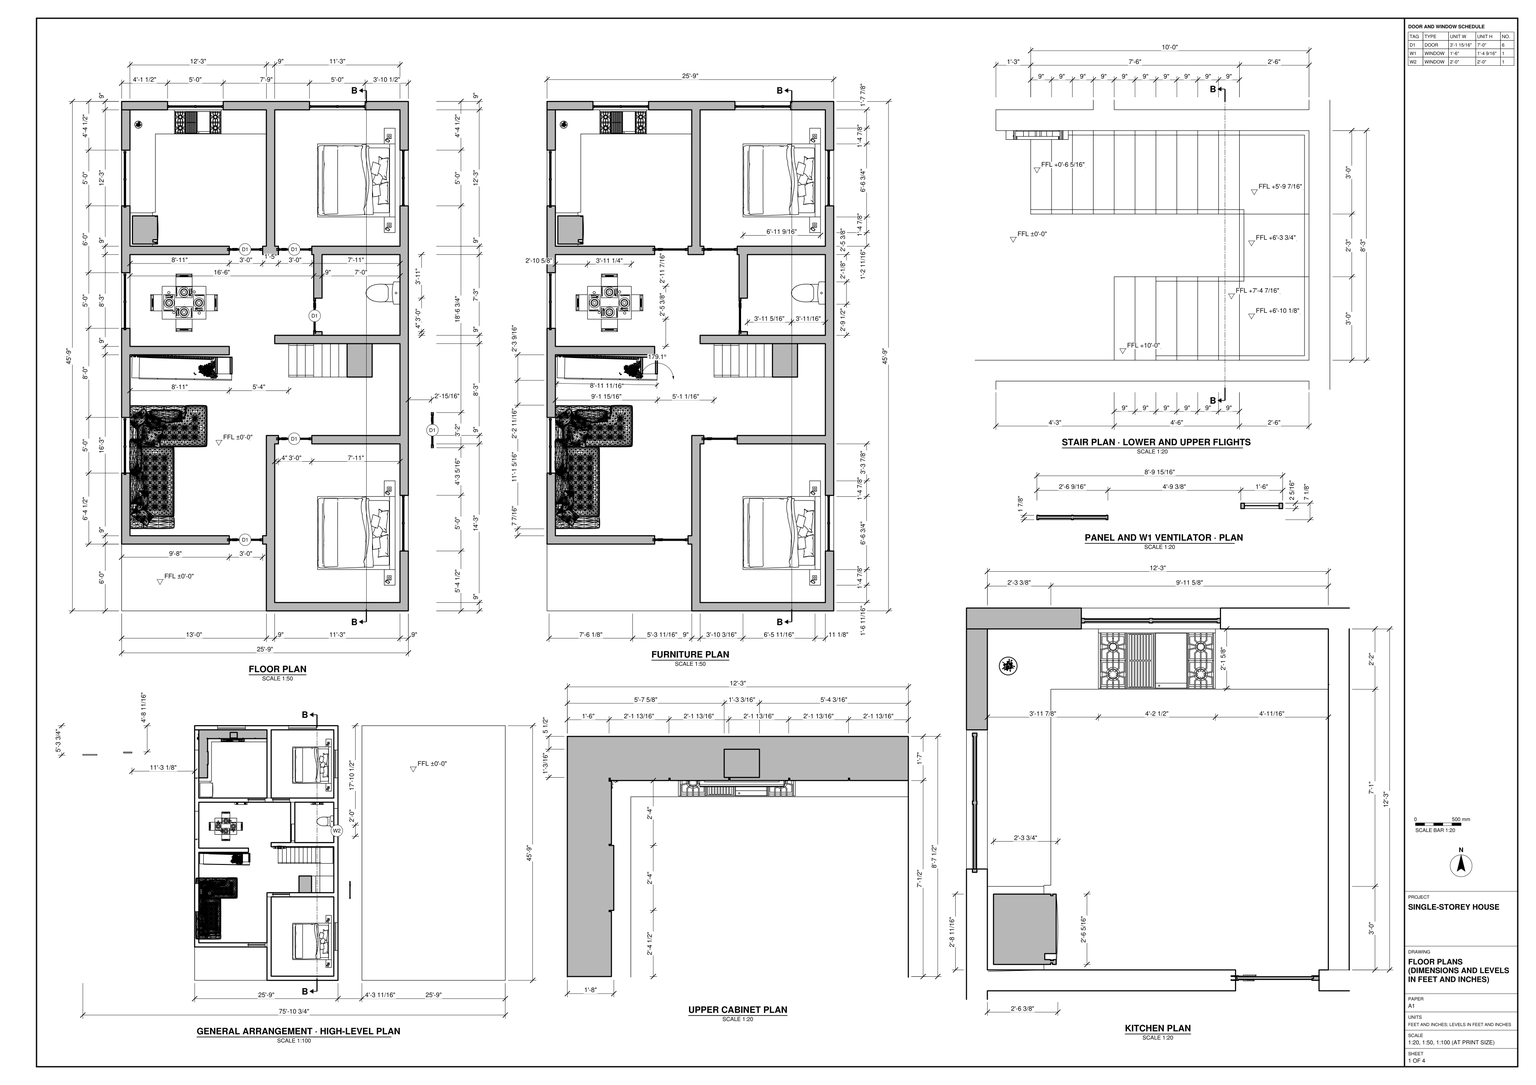
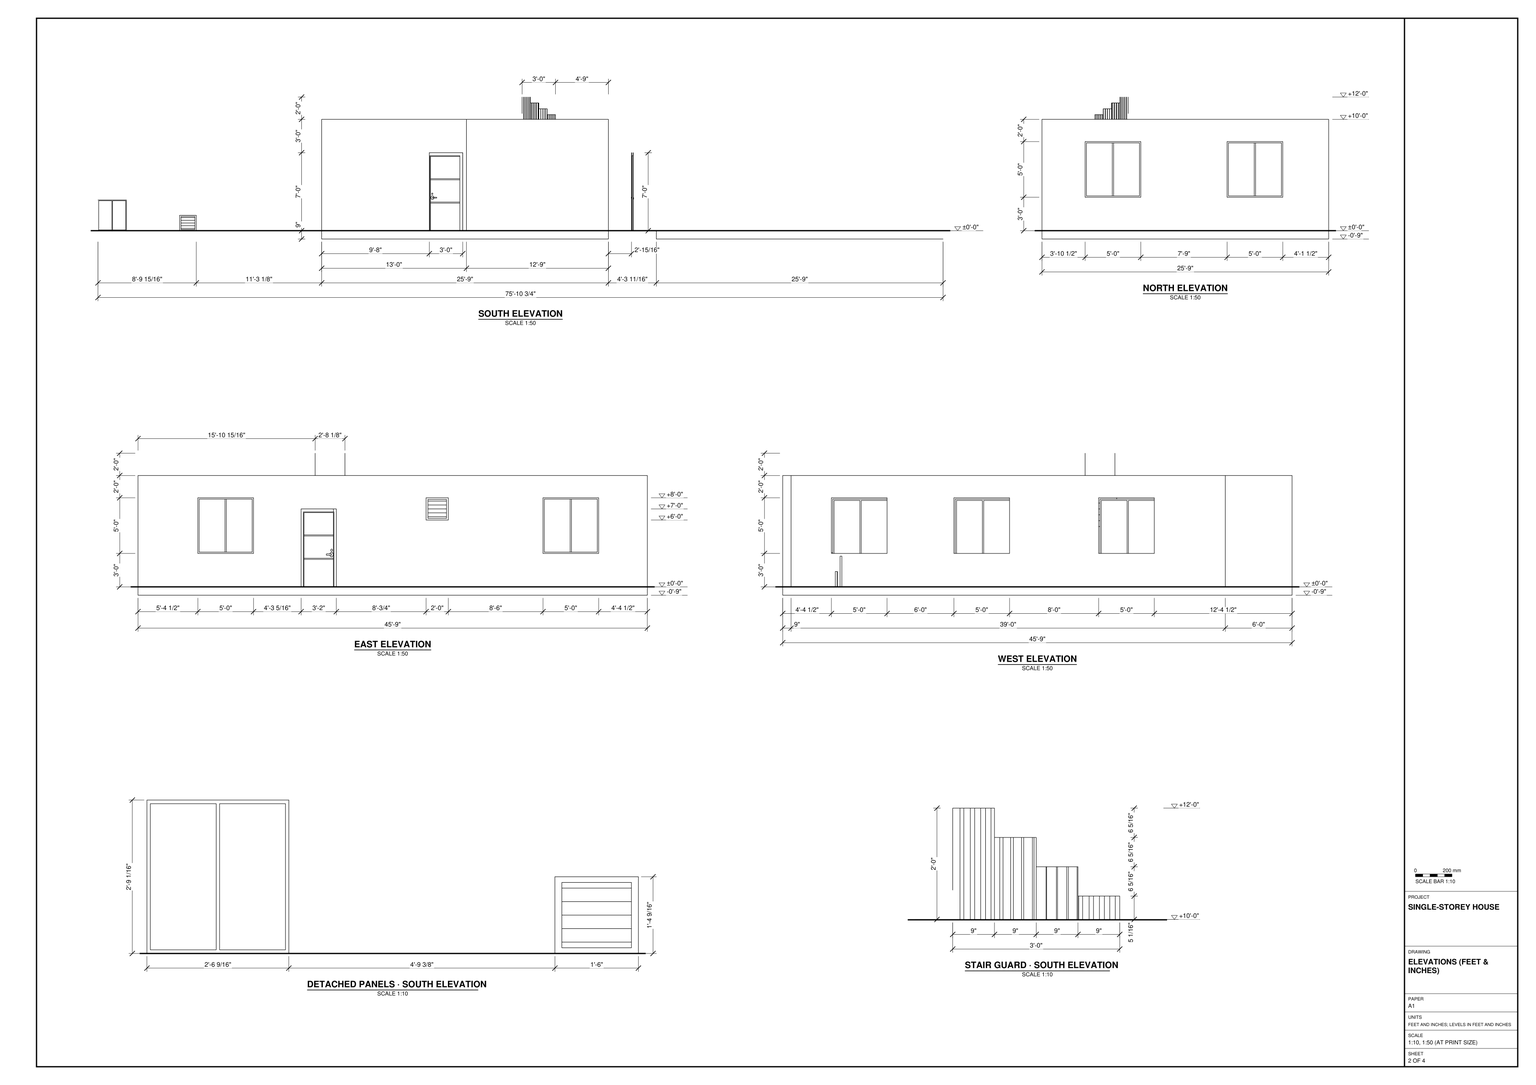
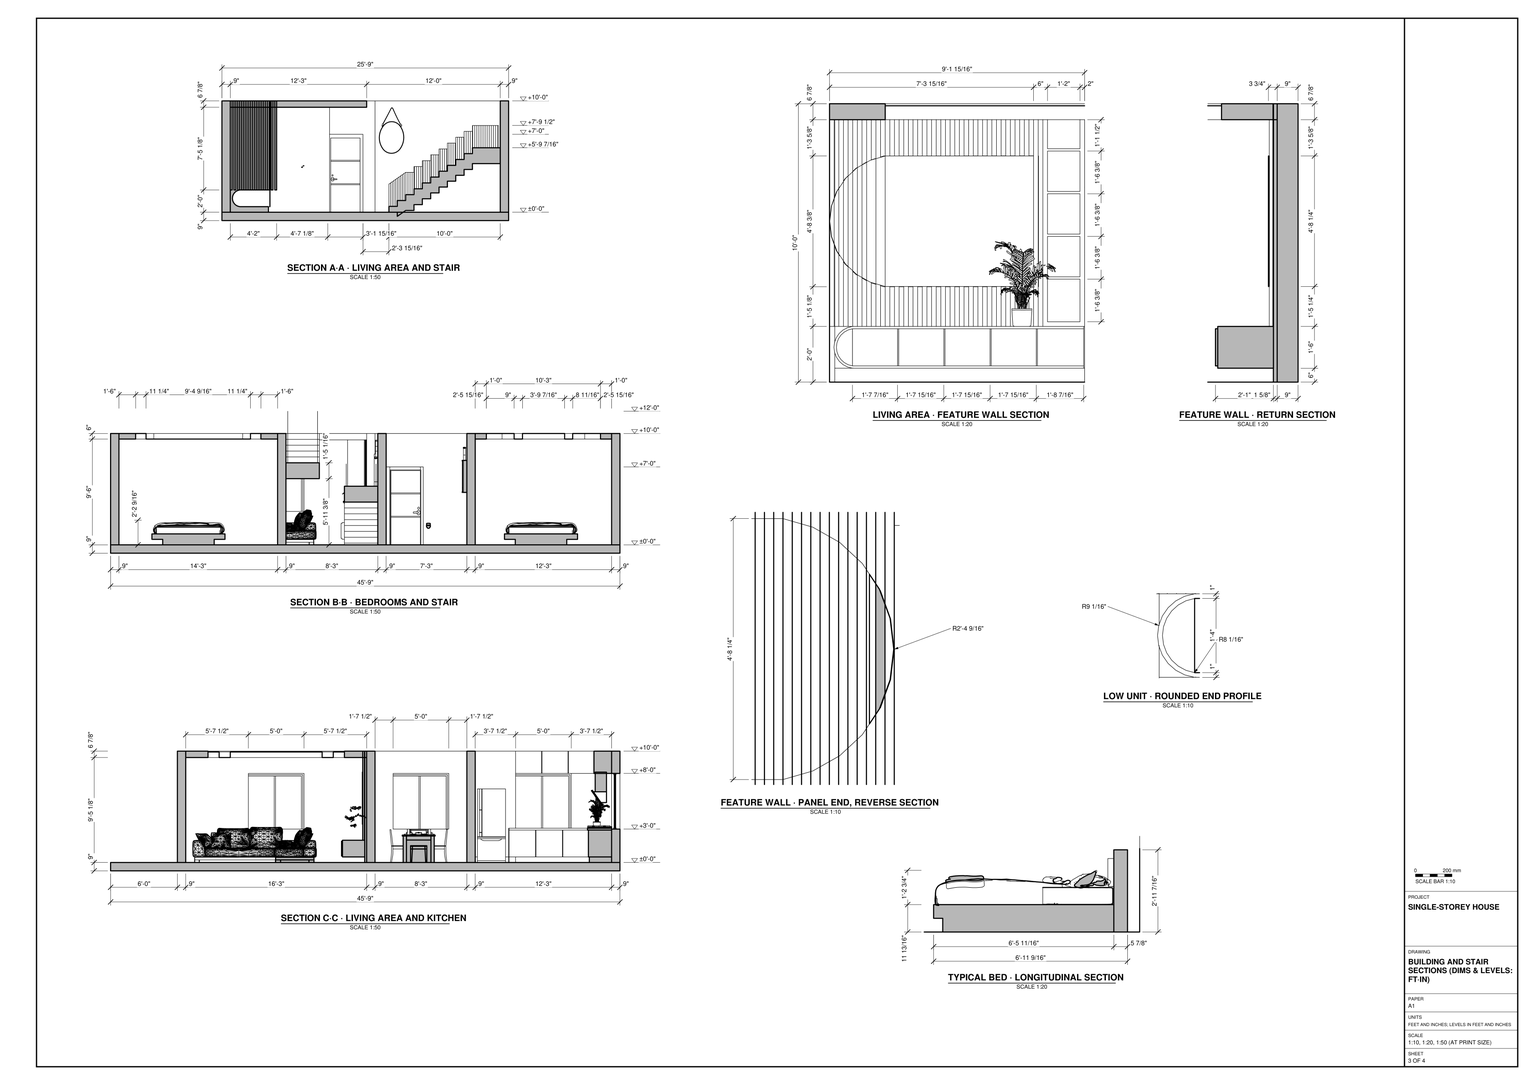
Build the single-storey house in SketchUp from task_files/diagram_01.pdf. Work in feet and inches. Set the ground-floor finished level to ±0'-0". The complete arrangement measures 75'-10 3/4" along X, 45'-9" along Y and 10'-9" along Z. The house itself is 25'-9" wide. Use the general arrangement plan to position the separate rectangular slab and detached units rather than widening the house to fill the overall extent.

Form the recessed southern entrance beside the projecting bedroom. Use the wall thicknesses shown on the floor plan, cut the door and window openings, and follow the sections for the slabs and roof. Place the kitchen in the northwest corner, with dining space immediately south of it and the living area by the entrance. Place the bedrooms at opposite ends of the east side, with the toilet compartment and return stair between them. Model both stair flights, the turning landing and the stepped guard.

Fit the kitchen with its L-shaped counter, upper cabinets, cooktop and hood. Use the furniture plan for the platform beds, four-place dining set and corner sofa. Reproduce the living-area feature wall, including the rounded panel end, low storage unit and side shelving. Decor and loose items may be any suitable library components. Keep shell elements and each furniture or joinery piece in separate groups or components, and use components for repeated parts. Save one SketchUp model as output_files/furnished_single_storey_house_with_a_return_stair.skp.

# SketchUp Ruby script. Lengths in inches.
U = 1.inch
M = Sketchup.active_model
def pt(a) = Geom::Point3d.new(a.map { |v| v * U })
def face(e, loops, mat)
  f = e.add_face(loops[0].map { |a| pt(a) })
  loops[1..].each { |l| e.add_face(l.map { |a| pt(a) }).erase! }
  f.material = f.back_material = mat if mat
  f
end
# faces: each face lists its corners as indices into pts; further lists are holes
def faces(e, pts, list, mat = nil) = list.each { |f| face(e, (f[0].is_a?(Array) ? f : [f]).map { |l| l.map { |i| pts[i] } }, mat) }
# xy, xz, yz: faces in a plane at the given z, y or x. An outline is a flat list of corners, or four numbers for a rectangle; further outlines are holes
def ring(l) = l.size == 4 ? [[l[0], l[1]], [l[2], l[1]], [l[2], l[3]], [l[0], l[3]]] : l.each_slice(2).to_a
def flat(e, list, mat, &to3) = list.each { |f| face(e, (f[0].is_a?(Array) ? f : [f]).map { |l| ring(l).map { |u, v| to3.(u, v) } }, mat) }
def xy(e, z, list, mat = nil) = flat(e, list, mat) { |x, y| [x, y, z] }
def xz(e, y, list, mat = nil) = flat(e, list, mat) { |x, z| [x, y, z] }
def yz(e, x, list, mat = nil) = flat(e, list, mat) { |y, z| [x, y, z] }
def lines(e, pts, list) = list.each { |a, b| e.add_line(pt(pts[a]), pt(pts[b])) }
# prism: a flat outline (further loops are holes) pulled along v
def prism(e, loops, v, mat = nil)
  f = face(e, loops, mat); d = Geom::Vector3d.new(v.map { |x| x * U })
  f.pushpull(f.normal.samedirection?(d) ? d.length : -d.length)
end
def box(e, o, s, mat = nil) = prism(e, [[o, [o[0] + s[0], o[1], o[2]], [o[0] + s[0], o[1] + s[1], o[2]], [o[0], o[1] + s[1], o[2]]]], [0, 0, s[2]], mat)
def at(x, y, z, deg = 0) = Geom::Transformation.translation(pt([x, y, z])) * Geom::Transformation.rotation(ORIGIN, Z_AXIS, deg.degrees)
def axes(o, x, y, z) = Geom::Transformation.new([*x, 0, *y, 0, *z, 0, *pt(o).to_a, 1])
def part(name) = M.definitions.add(name)
# library, detail: a bought-in or finely detailed component or shape, given as its bounding box
def library(name, o, s) = part(name).tap { |d| box(d.entities, o, s) }
def detail(e, o, s) = box(e.add_group.entities, o, s)
def put(e, d, t, mat = nil) = e.add_instance(d, t).tap { |i| i.material = mat if mat }
def group(e, t, mat = nil) = e.add_group.tap { |g| g.transformation = t; g.material = mat if mat }.entities
root = M.entities
M.materials.add("[0035_Tan]").color = [210, 180, 140]
M.materials.add("[0036_BurlyWood]").color = [222, 184, 135]
M.materials.add("[0042_Sienna]").color = [160, 82, 45]
M.materials.add("[0049_Beige]").color = [245, 245, 220]
M.materials.add("[0054_LightYellow]").color = [255, 255, 224]
M.materials.add("[0110_LightSlateGray]").color = [119, 136, 153]
M.materials.add("[0111_SlateGray]").color = [112, 128, 144]
M.materials.add("[0119_RosyBrown]").color = [188, 143, 143]
M.materials.add("[Carrera Marble]").color = [207, 207, 207]
M.materials["[Carrera Marble]"].alpha = 0.99
M.materials.add("[Color M09]").color = [0, 0, 0]
M.materials.add("[Color_008]").color = [30, 30, 30]
M.materials.add("[Color_009]").color = [0, 0, 0]
M.materials.add("[Translucent Glass Gray]").color = [128, 128, 128]
M.materials["[Translucent Glass Gray]"].alpha = 0.5
M.materials.add("[Translucent Glass Tinted]1").color = [7, 201, 240]
M.materials["[Translucent Glass Tinted]1"].alpha = 0.48
M.materials.add("[Translucent_Glass_Gray]").color = [128, 128, 128]
M.materials["[Translucent_Glass_Gray]"].alpha = 0.5
M.materials.add("[Wood Cherry Original]").color = [152, 86, 42]
M.materials.add("[Wood Floor Parquet]").color = [145, 89, 39]
M.materials.add("[Wood Floor]").color = [155, 105, 61]
c1 = library("main+door",[0,-0.79,0],[47.24,7.88,82.68])
c2 = part("ventilator")
g1 = group(c2.entities,at(0,0,0))
xy(g1,0,[[0,0,24,1],[0,1,24,6.83]],"[Wood Floor Parquet]")
xy(g1,1.75,[[2,0,22,6.83]],"[Wood Floor Parquet]")
xy(g1,21.87,[[2,0,22,6.83]],"[Wood Cherry Original]")
xy(g1,23.62,[[0,0,24,1],[0,1,24,6.83]],"[Wood Floor Parquet]")
xz(g1,0,[[[0,0,24,23.62],[2,1.75,22,21.87]]],"[Wood Floor Parquet]")
xz(g1,6.83,[[[0,0,24,23.62],[2,1.75,22,21.87]]],"[Wood Cherry Original]")
yz(g1,0,[[0,0,1,23.62],[1,0,6.83,23.62]],"[Wood Floor Parquet]")
yz(g1,2,[[0,1.75,6.83,1.75,6.83,7.66,0,3.5],[0,3.5,6.83,7.66,6.83,11.8125,0,7.66],[0,7.66,6.83,11.8125,6.83,15.97,0,11.8125],[0,11.8125,6.83,15.97,6.83,20.12,0,15.97],[0,15.97,6.83,20.12,6.83,21.87,0,21.87]],"[Wood Floor Parquet]")
yz(g1,22,[[0,1.75,0,3.5,6.83,7.66,6.83,1.75],[0,3.5,0,7.66,6.83,11.8125,6.83,7.66],[0,7.66,0,11.8125,6.83,15.97,6.83,11.8125],[0,11.8125,0,15.97,6.83,20.12,6.83,15.97],[0,15.97,0,21.87,6.83,21.87,6.83,20.12]],"[Wood Floor Parquet]")
yz(g1,24,[[0,0,1,23.62],[1,0,6.83,23.62]],"[Wood Floor Parquet]")
p = [[2,0,3.5],[2,6.83,7.66],[22,6.83,7.66],[22,0,3.5],[2,6.83,11.8125],[2,0,7.66],
  [22,0,7.66],[22,6.83,11.8125],[2,0,11.8125],[2,6.83,15.97],[22,6.83,15.97],[22,0,11.8125],
  [2,6.83,20.12],[2,0,15.97],[22,0,15.97],[22,6.83,20.12]]
faces(g1,p,[[0,1,2,3],[4,5,6,7],[8,9,10,11]],"[Translucent Glass Tinted]1")
faces(g1,p,[[12,13,14,15]],"[Translucent Glass Gray]")
c3 = library("Component\#33",[0,0,0],[60.64,55.48,158.625])
c4 = library("Gas cooktop",[0,0,34.52],[24.41,48.07,2.63])
c5 = part("Inclined chimney")
g2 = group(c5.entities,at(1.97,2.08,2.89))
xy(g2,0,[[0,7.9,31.3,13.68]])
xy(g2,11.29,[[0,0,31.3,13.68]])
xz(g2,13.68,[[0,0,31.3,11.29]])
yz(g2,0,[[7.9,0,0,11.29,13.68,11.29,13.68,0]])
yz(g2,31.3,[[7.9,0,13.68,0,13.68,11.29,0,11.29]])
g3 = group(c5.entities,at(0,9.85,0.4))
g4 = group(g3,at(0,0.61,0.43))
prism(g4,[[[35.24,0,0],[35.24,-3.39,4.84],[35.24,-3.58,4.7],[35.24,-0.29,0]]],[-35.24,0,0])
g5 = group(g3,at(0,-3.21,4.99))
prism(g5,[[[35.24,-0.2,-0.12],[35.24,-3.16,5],[0,-3.16,5],[0,-0.2,-0.12]]],[0,0.2,0.12])
g6 = group(g3,at(0,-6.27,10.27))
prism(g6,[[[35.24,-0.19,-0.14],[35.24,-3.58,4.7],[0,-3.58,4.7],[0,-0.19,-0.14]]],[0,0.19,0.14])
g7 = group(g3,at(0,0.61,0.43))
prism(g7,[[[35.24,0,0],[35.24,0.96,0],[35.24,-9.52,14.96],[35.24,-10.16,14.51]]],[-35.24,0,0])
g8 = group(c5.entities,at(10.24,3.95,20.8))
box(g8,[0,0,-6.62],[14.76,11.8125,20.56])
g9 = group(c5.entities,at(0,10.1,0))
prism(g9,[[[35.24,0.46,0],[35.24,1.33,0],[35.24,1.33,0.83],[35.24,1.01,0.83],[35.24,0.37,0.83],[35.24,0,0.83],[35.24,0,0.64]]],[-35.24,0,0])
c6 = part("Inclined+chimney")
put(c6.entities,c5,at(34.17,38.97,0.69))
c7 = library("Double bed",[0,0,0],[83.59,112.46,35.43])
c8 = library("CS300DRT",[0,0,0],[27.18,17.85,30.31])
c9 = library("Senza",[-40.91,-66.2,-0.5],[133.3,90.15,38.26])
c10 = library("SKT_Nearly Natural 5' Kentia Palm Silk Tree",[-23.18,-17.61,0],[47.48,43.95,59.125])
c11 = library("DINING+TABLE_4+SEATER_+1200mm+x+900mm",[14.07,13.24,0],[72.26,62.1,36.02])
c12 = library("Round wall hanging",[0,0,0],[26.88,1.18,49.49])
c13 = part("Group\#2")
xy(c13.entities,0,[[0,0,82.68,1.18]],"[Color_009]")
xy(c13.entities,1.97,[[1.97,0.98,40.35,1.18],[42.32,0.98,80.71,1.18]])
xy(c13.entities,1.97,[[1.97,0,40.35,0.3],[42.32,0,80.71,0.3]],"[Color_009]")
xy(c13.entities,80.71,[[1.97,0,40.35,0.3],[42.32,0,80.71,0.3],[1.97,0.3,40.35,0.98],[42.32,0.3,80.71,0.98],[1.97,0.98,40.35,1.18],
  [42.32,0.98,80.71,1.18]])
xy(c13.entities,82.68,[[0,0,82.68,1.18]],"[Color_008]")
xz(c13.entities,0,[[[0,0,82.68,82.68],[1.97,1.97,40.35,80.71],[42.32,1.97,80.71,80.71]]],"[Color_009]")
xz(c13.entities,0.3,[[1.97,1.97,40.35,80.71],[42.32,1.97,80.71,80.71]],"[Translucent_Glass_Gray]")
xz(c13.entities,0.98,[[1.97,1.97,40.35,80.71],[42.32,1.97,80.71,80.71]],"[Translucent_Glass_Gray]")
xz(c13.entities,1.18,[[[0,0,82.68,82.68],[1.97,1.97,80.71,80.71]],[40.35,1.97,42.32,80.71]],"[Color_009]")
yz(c13.entities,0,[[0,0,1.18,82.68]],"[Color_009]")
yz(c13.entities,1.97,[[0.98,1.97,1.18,80.71]])
yz(c13.entities,1.97,[[0,1.97,0.3,80.71]],"[Color_009]")
yz(c13.entities,40.35,[[0,1.97,0.3,80.71],[0.98,1.97,1.18,80.71]],"[Color_009]")
yz(c13.entities,42.32,[[0,1.97,0.3,80.71],[0.98,1.97,1.18,80.71]])
yz(c13.entities,80.71,[[0,1.97,0.3,80.71],[0.98,1.97,1.18,80.71]],"[Color_009]")
yz(c13.entities,82.68,[[0,0,1.18,82.68]],"[Color_009]")
c14 = library("Group\#5",[0,0,-4.44],[120,99,148.43])
c15 = part("Square post")
box(c15.entities,[0,-2,0],[2,2,96])
c16 = part("Group\#8")
box(c16.entities,[0,-2,0],[2,2,96])
xy(root,0,[[274.45,516,397.07,540]])
xy(root,6,[[274.95,515,298.97,516],[299.47,515,323.5,516],[324,515,348.02,516],[348.52,515,372.55,516],[373.05,515,396.87,516]])
xy(root,34.9375,[[274.95,515,298.97,515,298.97,516,299.47,516,299.47,515,323.5,515,323.5,516,324,516,324,515,348.02,515,348.02,516,348.52,516,348.52,515,372.55,515,372.55,516,373.05,516,373.05,515,396.87,515,396.87,516,397.07,516,397.07,540,274.45,540,274.45,516,274.95,516]])
xy(root,96,[[250.07,436.5,250.07,540,268.07,540,268.07,520.69,269.07,520.69,269.07,493.5,268.07,493.5,268.07,493,270.07,493,270.07,465,268.07,465,268.07,464.5,269.07,464.5,269.07,436.5],[268.57,521,268.57,522,268.07,522,268.07,540,397.07,540,397.07,521,371.77,521,371.77,522,371.27,522,371.27,521,345.97,521,345.97,522,345.47,522,345.47,521,320.17,521,320.17,522,319.67,522,319.67,521,294.37,521,294.37,522,293.87,522,293.87,521]])
xy(root,120,[[250.07,436.5,269.07,436.5,269.07,464.5,268.07,464.5,268.07,465,270.07,465,270.07,493,268.07,493,268.07,493.5,269.07,493.5,269.07,520.69,268.07,520.69,268.07,540,250.07,540],[268.57,521,293.87,521,293.87,522,294.37,522,294.37,521,319.67,521,319.67,522,320.17,522,320.17,521,345.47,521,345.47,522,345.97,522,345.97,521,371.27,521,371.27,522,371.77,522,371.77,521,397.07,521,397.07,540,268.07,540,268.07,522,268.57,522]],"[Wood Floor]")
xz(root,436.5,[[250.07,96,269.07,120]],"[Wood Floor]")
xz(root,464.5,[[268.07,96,269.07,120]],"[Wood Floor]")
xz(root,465,[[268.07,96,270.07,120]],"[Wood Floor]")
xz(root,493,[[268.07,96,270.07,120]],"[Wood Floor]")
xz(root,493.5,[[268.07,96,269.07,120]],"[Wood Floor]")
xz(root,515,[[274.95,6,298.97,34.9375],[299.47,6,323.5,34.9375],[324,6,348.02,34.9375],[348.52,6,372.55,34.9375],[373.05,6,396.87,34.9375]],"[Wood Floor]")
xz(root,516,[[274.45,0,274.95,34.9375],[274.95,0,397.07,0,397.07,34.9375,396.87,34.9375,396.87,6,373.05,6,373.05,34.9375,372.55,34.9375,372.55,6,348.52,6,348.52,34.9375,348.02,34.9375,348.02,6,324,6,324,34.9375,323.5,34.9375,323.5,6,299.47,6,299.47,34.9375,298.97,34.9375,298.97,6,274.95,6],[397.07,0,397.57,34.9375]])
xz(root,520.69,[[268.07,96,269.07,120]],"[Wood Floor]")
xz(root,521,[[268.57,96,293.87,120],[294.37,96,319.67,120],[320.17,96,345.47,120],[345.97,96,371.27,120],[371.77,96,397.07,120]],"[Wood Floor]")
xz(root,522,[[268.07,96,268.57,120],[293.87,96,294.37,120],[319.67,96,320.17,120],[345.47,96,345.97,120],[371.27,96,371.77,120]])
xz(root,540,[[274.45,0,397.07,34.9375]])
yz(root,250.07,[[436.5,96,540,120]])
yz(root,268.07,[[464.5,96,465,120],[493,96,493.5,120],[520.69,96,522,120]],"[Wood Floor]")
yz(root,268.57,[[521,96,522,120]])
yz(root,269.07,[[436.5,96,464.5,120],[493.5,96,520.69,120]],"[Wood Floor]")
yz(root,270.07,[[465,96,493,120]],"[Wood Floor]")
yz(root,274.45,[[516,0,540,34.9375]])
yz(root,274.95,[[515,6,516,34.9375]])
yz(root,293.87,[[521,96,522,120]])
yz(root,294.37,[[521,96,522,120]])
yz(root,298.97,[[515,6,516,34.9375]])
yz(root,299.47,[[515,6,516,34.9375]])
yz(root,319.67,[[521,96,522,120]])
yz(root,320.17,[[521,96,522,120]])
yz(root,323.5,[[515,6,516,34.9375]])
yz(root,324,[[515,6,516,34.9375]])
yz(root,345.47,[[521,96,522,120]])
yz(root,345.97,[[521,96,522,120]])
yz(root,348.02,[[515,6,516,34.9375]])
yz(root,348.52,[[515,6,516,34.9375]])
yz(root,371.27,[[521,96,522,120]])
yz(root,371.77,[[521,96,522,120]])
yz(root,372.55,[[515,6,516,34.9375]])
yz(root,373.05,[[515,6,516,34.9375]])
yz(root,396.87,[[515,6,516,34.9375]])
yz(root,397.07,[[516,0,540,34.9375],[521,96,540,120]])
# 242 loose lines left out
put(root,c1,axes([574.98,213.76,0],[0,-0.80367,0],[0.33,0,0],[0,0,1.016]))
put(root,c2,axes([87.9375,490.01,0],[0.75,0,0],[0,0.34,0],[0,0,0.7]))
put(root,c3,axes([280.47,395.36,0],[0,0.5,0],[-0.5,0,0],[0,0,0.5]))
put(root,c4,axes([297.92,540,0.69],[0,-1.05,0],[1.05,0,0],[0,0,1.05]))
put(root,c6,axes([271.95,478.09,60.89],[1.03,0,0],[0,1.03,0],[0,0,1.03]))
put(root,c7,at(452.24,407.69,0))
put(root,c7,at(452.24,27.69,0))
put(root,c8,axes([541.07,354.625,0],[-1.35,0,0],[0,-1.35,0],[0,0,1.35]))
put(root,c9,at(267.2,129.36,0.5,90))
put(root,c10,axes([332.98,259.47,24],[0.66,0,0],[0,0.66,0],[0,0,0.66]))
put(root,c11,at(258.14,287.78,0))
put(root,c12,axes([410.43,284.14,63.26],[1,0,0],[0,4.27,0],[0,0,1]))
put(root,c10,axes([259.04,523.94,36.9375],[0.6,0,0],[0,0.6,0],[0,0,0.6]))
put(root,c12,axes([327.71,378.96,62.07],[1,0,0],[0,4.27,0],[0,0,1]))
put(root,c12,axes([492.11,378.96,56.46],[1,0,0],[0,4.27,0],[0,0,1]))
put(root,c13,axes([0,485.22,0],[0.37,0,0],[0,1.625,0],[0,0,0.4]))
g10 = group(root,at(241.07,0,0),"[0119_RosyBrown]")
xy(g10,0,[[156,0,156,180,165,180,165,9,300,9,300,124.5,309,124.5,309,0],[0,72,0,148.5,9,148.5,9,81,116,81,116,72],[152,72,156,81],[300,124.5,300,180,205,180,205,189,300,189,300,288,165,288,165,297,300,297,300,370.5,309,370.5,309,124.5],[0,148.5,0,304.5,9,304.5,9,285,116,285,116,276,9,276,9,148.5],
  [156,180,169,189],[207,297,216,301],[0,304.5,0,436.5,9,436.5,9,393,116,393,116,384,9,384,9,304.5],[207,337,216,384],[300,370.5,300,384,205,384,205,393,300,393,300,496.5,309,496.5,309,370.5],
  [152,384,169,393],[156,393,156,540,49.5,540,49.5,549,202.5,549,202.5,540,165,540,165,393],[9,429,9,540,33.875,540,33.875,516,33.375,516,33.375,429],[0,436.5,9,540],[300,496.5,300,540,202.5,540,202.5,549,309,549,309,496.5],
  [0,540,49.5,549]])
xy(g10,6,[[33.375,429.5,34.375,458],[33.375,458.5,34.375,487],[33.375,487.5,34.375,514.75]])
xy(g10,34.9375,[[33.375,429.5,34.375,458],[34.375,429.5,36.375,458],[33.375,458,36.375,458.5],[33.375,458.5,34.375,487],[34.375,458.5,36.375,487],
  [33.375,487,36.375,487.5],[33.375,487.5,34.375,487.5,34.375,514,33.875,514,33.875,514.75,33.375,514.75],[34.375,487.5,36.375,514],[33.875,514,34.375,514.75],[34.375,514,34.375,514.75,33.875,514.75,33.875,540,156,540,156,514]])
xy(g10,36,[[300,64.5,309,124.5],[0,148.5,9,208.5],[0,304.5,9,364.5],[0,436.5,9,496.5],[300,436.5,309,496.5],
  [49.5,540,109.5,549],[202.5,540,262.5,549]])
xy(g10,36.9375,[[9,429,33.375,429,33.375,429.5,36.375,429.5,36.375,514,156,514,156,540,9,540]],"[Carrera Marble]")
xy(g10,72,[[300,310.5,309,334.5]])
xy(g10,84,[[116,72,152,81],[169,180,205,189],[207,301,216,337],[116,384,152,393],[169,384,205,393]])
xy(g10,96,[[300,64.5,309,124.5],[0,148.5,9,208.5],[0,304.5,9,364.5],[300,310.5,309,334.5],[0,436.5,9,496.5],
  [300,436.5,309,496.5],[49.5,540,109.5,549],[202.5,540,262.5,549]])
xy(g10,120,[[[156,0,309,0,309,549,0,549,0,540,156,540,156,393,9,393,9,540,0,540,0,72,156,72],[9,81,9,276,116,276,116,285,9,285,9,384,207,384,207,297,165,297,165,288,300,288,300,189,156,189,156,81],[165,9,300,180],[165,393,300,540],[216,297,300,384]]])
xz(g10,0,[[156,0,309,120]],"[0049_Beige]")
xz(g10,9,[[165,0,300,120]])
xz(g10,64.5,[[300,36,309,96]])
xz(g10,72,[[0,0,116,0,116,84,152,84,152,0,156,0,156,120,0,120]],"[0110_LightSlateGray]")
xz(g10,81,[[9,0,9,120,156,120,156,0,152,0,152,84,116,84,116,0]])
xz(g10,124.5,[[300,36,309,96]])
xz(g10,148.5,[[0,36,9,96]])
xz(g10,180,[[165,0,169,0,169,84,205,84,205,0,300,0,300,120,165,120]])
xz(g10,189,[[156,0,156,120,300,120,300,0,205,0,205,84,169,84,169,0]],"[0035_Tan]")
xz(g10,208.5,[[0,36,9,96]])
xz(g10,276,[[9,0,116,120]])
xz(g10,285,[[9,0,116,120]],"[0035_Tan]")
xz(g10,288,[[165,0,300,120]])
xz(g10,297,[[207,0,216,84]])
xz(g10,297,[[165,0,207,120],[216,0,300,120]],"[0035_Tan]")
xz(g10,301,[[207,0,216,84]])
xz(g10,304.5,[[0,36,9,96]])
xz(g10,310.5,[[300,72,309,96]])
xz(g10,334.5,[[300,72,309,96]])
xz(g10,337,[[207,0,216,84]])
xz(g10,364.5,[[0,36,9,96]])
xz(g10,384,[[216,0,300,120]],"[0110_LightSlateGray]")
xz(g10,384,[[9,0,116,0,116,84,152,84,152,0,169,0,169,84,205,84,205,0,207,0,207,120,9,120]],"[0111_SlateGray]")
xz(g10,393,[[9,0,9,120,156,120,156,0,152,0,152,84,116,84,116,0],[165,0,165,120,300,120,300,0,205,0,205,84,169,84,169,0]])
xz(g10,429,[[9,0,33.375,36.9375]])
xz(g10,429.5,[[33.375,6,34.375,34.9375],[33.375,34.9375,36.375,36.9375]])
xz(g10,436.5,[[0,36,9,96],[300,36,309,96]])
xz(g10,458,[[33.375,6,34.375,34.9375]])
xz(g10,458.5,[[33.375,6,34.375,34.9375]])
xz(g10,487,[[33.375,6,34.375,34.9375]])
xz(g10,487.5,[[33.375,6,34.375,34.9375]])
xz(g10,496.5,[[0,36,9,96],[300,36,309,96]])
xz(g10,514,[[36.375,34.9375,156,36.9375]],"[Carrera Marble]")
xz(g10,514.75,[[33.375,6,34.375,34.9375]])
xz(g10,540,[[0,0,9,120],[9,0,33.875,36.9375],[33.875,0,156,34.9375],[[165,0,300,120],[202.5,36,262.5,96]],[33.875,34.9375,156,34.9375,156,36.9375,109.5,36.9375,109.5,36,49.5,36,49.5,36.9375,33.875,36.9375],
  [49.5,36,109.5,36.9375],[9,36.9375,49.5,36.9375,49.5,96,109.5,96,109.5,36.9375,156,36.9375,156,120,9,120]])
xz(g10,549,[[[0,0,309,120],[202.5,36,262.5,96],[49.5,36,109.5,96]]],"[0049_Beige]")
yz(g10,0,[[540,0,549,120]])
yz(g10,0,[[[72,0,540,120],[304.5,36,364.5,96],[436.5,36,496.5,96],[148.5,36,208.5,96]]],"[0049_Beige]")
yz(g10,9,[[[81,0,276,120],[148.5,36,208.5,96]],[393,0,429,0,429,36.9375,436.5,36.9375,436.5,96,496.5,96,496.5,36.9375,540,36.9375,540,120,393,120],[429,0,436.5,36.9375],[436.5,0,540,0,540,36.9375,496.5,36.9375,496.5,36,436.5,36],[436.5,36,496.5,36.9375]])
yz(g10,9,[[[285,0,384,120],[304.5,36,364.5,96]]],"[0049_Beige]")
yz(g10,33.375,[[429,0,429.5,34.9375],[429.5,6,458,34.9375],[458.5,6,487,34.9375],[487.5,6,514.75,34.9375],[429,34.9375,429.5,36.9375]])
yz(g10,33.875,[[516,0,540,34.9375]])
yz(g10,34.375,[[429.5,6,458,34.9375],[458.5,6,487,34.9375],[487.5,6,514.75,34.9375]],"[Wood Floor]")
yz(g10,36.375,[[429.5,34.9375,514,36.9375]])
yz(g10,49.5,[[540,36,549,96]])
yz(g10,109.5,[[540,36,549,96]])
yz(g10,116,[[72,0,81,84],[276,0,285,120],[384,0,393,84]])
yz(g10,152,[[72,0,81,84],[384,0,393,84]])
yz(g10,156,[[0,0,72,120],[81,0,189,120],[514,34.9375,540,36.9375]])
yz(g10,156,[[393,0,393,120,540,120,540,36.9375,514,36.9375,514,34.9375,540,34.9375,540,0]],"[0054_LightYellow]")
yz(g10,165,[[9,0,180,120],[288,0,297,120],[393,0,540,120]])
yz(g10,169,[[180,0,189,84],[384,0,393,84]])
yz(g10,202.5,[[540,36,549,96]])
yz(g10,205,[[180,0,189,84],[384,0,393,84]])
yz(g10,207,[[297,0,297,120,384,120,384,0,337,0,337,84,301,84,301,0]],"[0054_LightYellow]")
yz(g10,216,[[297,0,301,84]])
yz(g10,216,[[337,0,384,0,384,120,297,120,297,84,337,84]],"[0049_Beige]")
yz(g10,262.5,[[540,36,549,96]])
yz(g10,300,[[[9,0,180,120],[64.5,36,124.5,96]],[189,0,288,120],[[393,0,540,120],[436.5,36,496.5,96]]])
yz(g10,300,[[[297,0,384,120],[310.5,72,334.5,96]]],"[0035_Tan]")
yz(g10,309,[[[0,0,549,120],[436.5,36,496.5,96],[64.5,36,124.5,96],[310.5,72,334.5,96]]],"[0049_Beige]")
# 7 loose lines left out
put(g10,c1,axes([167.1,388.51,0],[0.80367,0,0],[0,0.33,0],[0,0,1.016]))
put(g10,c2,axes([305.35,334.5,72],[0,-1,0],[0.34,0,0],[0,0,1.016]))
put(g10,c1,axes([114.1,388.51,0],[0.80367,0,0],[0,0.33,0],[0,0,1.016]))
put(g10,c1,axes([207,337,0],[0,-0.80367,0],[0.33,0,0],[0,0,1.016]))
put(g10,c1,axes([167.03,184.5,0],[0.80367,0,0],[0,0.33,0],[0,0,1.016]))
put(g10,c1,axes([114.1,75.64,0],[0.80367,0,0],[0,0.33,0],[0,0,1.016]))
put(g10,c13,axes([202.5,542.58,36],[0.72571,0,0],[0,1.625,0],[0,0,0.72571]))
put(g10,c13,axes([302.58,496.5,36],[0,-0.72571,0],[1.625,0,0],[0,0,0.72571]))
put(g10,c13,axes([49.5,542.58,36],[0.72571,0,0],[0,1.625,0],[0,0,0.72571]))
put(g10,c13,axes([2.58,363.07,34.57],[0,-0.72571,0],[1.625,0,0],[0,0,0.72571]))
put(g10,c13,axes([2.58,207.07,34.57],[0,-0.72571,0],[1.625,0,0],[0,0,0.72571]))
put(g10,c13,axes([302.58,124.5,36],[0,-0.72571,0],[1.625,0,0],[0,0,0.72571]))
put(g10,c13,axes([2.58,495.07,34.57],[0,-0.72571,0],[1.625,0,0],[0,0,0.72571]))
g11 = group(root,at(241.07,0,-9))
box(g11,[0,0,0],[309,549,9],"[Carrera Marble]")
put(root,c14,at(421.07,189,0))
g12 = group(root,at(250.07,248.42,0))
xy(g12,24,[[91.96,7,109.96,25]])
xy(g12,26,[[93.96,7,107.96,25]],"[Wood Floor]")
xy(g12,44.4,[[93.96,7,107.96,25]])
xy(g12,45.4,[[93.96,7,107.96,25]],"[Wood Floor]")
xy(g12,62.8,[[93.96,7,107.96,25]])
xy(g12,63.8,[[93.96,7,107.96,25]],"[Wood Floor]")
xy(g12,81.2,[[93.96,7,107.96,25]])
xy(g12,82.2,[[93.96,7,107.96,25]],"[Wood Floor]")
xy(g12,99.6,[[93.96,7,107.96,25]])
xy(g12,100.6,[[93.96,7,107.96,25]],"[Wood Floor]")
xy(g12,118,[[93.96,7,107.96,25]])
xy(g12,120,[[91.96,7,109.96,25]])
xz(g12,7,[[[91.96,24,109.96,120],[93.96,26,107.96,44.4],[93.96,63.8,107.96,81.2],[93.96,100.6,107.96,118],[93.96,82.2,107.96,99.6],[93.96,45.4,107.96,62.8]]],"[Color M09]")
xz(g12,25,[[[91.96,24,109.96,120],[93.96,26,107.96,44.4],[93.96,63.8,107.96,81.2],[93.96,100.6,107.96,118],[93.96,82.2,107.96,99.6],[93.96,45.4,107.96,62.8]]])
xz(g12,25,[[93.96,26,107.96,44.4],[93.96,45.4,107.96,62.8],[93.96,63.8,107.96,81.2],[93.96,82.2,107.96,99.6],[93.96,100.6,107.96,118]],"[Wood Floor]")
yz(g12,91.96,[[7,24,25,120]])
yz(g12,93.96,[[7,26,25,44.4],[7,45.4,25,62.8],[7,63.8,25,81.2],[7,82.2,25,99.6],[7,100.6,25,118]],"[Wood Floor]")
yz(g12,107.96,[[7,26,25,44.4],[7,45.4,25,62.8],[7,63.8,25,81.2],[7,82.2,25,99.6],[7,100.6,25,118]],"[Wood Floor]")
yz(g12,109.96,[[7,24,25,120]])
# 5 loose lines left out
p = [[0,27.58,0],[0,27.58,24],[2.25,26.71,24],[2.25,26.71,0]]
faces(g12,p,[[0,1,2,3]])
put(g12,c15,at(87.96,25,24),"[0110_LightSlateGray]")
put(g12,c16,at(79.97,25.23,24),"[0110_LightSlateGray]")
put(g12,c16,at(63.97,25.7,24),"[0110_LightSlateGray]")
put(g12,c16,at(75.97,25.35,24),"[0110_LightSlateGray]")
put(g12,c16,at(71.97,25.47,24),"[0110_LightSlateGray]")
put(g12,c16,at(59.97,25.82,24),"[0110_LightSlateGray]")
put(g12,c16,at(55.98,25.9375,24),"[0110_LightSlateGray]")
put(g12,c16,at(51.98,26.05,24),"[0110_LightSlateGray]")
put(g12,c16,at(47.98,26.17,24),"[0110_LightSlateGray]")
put(g12,c16,at(83.96,25.11,24),"[0110_LightSlateGray]")
put(g12,c16,at(67.97,25.58,24),"[0110_LightSlateGray]")
put(g12,c16,at(43.98,26.29,24),"[0110_LightSlateGray]")
put(g12,c16,at(19.99,26.99,24),"[0110_LightSlateGray]")
g13 = group(g12,at(0,0,0),"[0049_Beige]")
p = [[6.6,25.79,87.61],[3,25.68,82.07],[17.0625,26.125,95.53],[11.37,25.94,92.17],[23.36,26.33,97.49],[0.76,25.61,75.86],
  [0,25.58,69.3],[6.6,25.79,50.99],[11.37,25.94,46.43],[17.0625,26.125,43.07],[23.36,26.33,41.11],[0.76,25.61,62.74],
  [3,25.68,56.53]]
lines(g13,p,[[0,1],[2,3],[4,2],[1,5],[3,0],[5,6],[7,8],[9,10],[6,11],[8,9],[11,12],[12,7]])
g14 = group(g13,at(2.25,25,0),"[0049_Beige]")
xy(g14,0,[[107.71,-0.03,0,1.71,0,1.74,107.71,0]])
xy(g14,6,[[107.32,-24,7.64,-22.39,8.03,1.58,107.71,-0.03]])
xy(g14,7,[[107.31,-25,87.37,-24.67,87.39,-23.67,107.32,-24],[86.87,-24.67,67.44,-24.34,67.45,-23.35,86.89,-23.67],[66.9375,-24.34,47.5,-24.01,47.52,-23.03,67.45,-23.35,66.95,-23.35],[47,-24.01,27.5625,-23.68,27.58,-22.71,47.52,-23.03,47.02,-23.03],[27.0625,-23.68,7.63,-23.35,7.64,-22.39,27.58,-22.71,27.08,-22.71]])
xy(g14,23,[[107.31,-25,107.32,-24,87.39,-23.67,87.37,-24.67],[86.87,-24.67,86.89,-23.67,67.45,-23.35,67.44,-24.34],[66.9375,-24.34,66.95,-23.35,67.45,-23.35,47.52,-23.03,47.5,-24.01],[47,-24.01,47.02,-23.03,47.52,-23.03,27.58,-22.71,27.5625,-23.68],[27.0625,-23.68,27.08,-22.71,7.64,-22.39,7.63,-23.35]])
xy(g14,24,[[107.32,-24,107.71,0,89.71,0,8.03,1.58,0,1.74,0,1.71,8.03,1.58,7.64,-22.39],[89.71,0,107.71,0,0,1.74,8.03,1.58]])
xy(g14,120,[[89.71,0,0,1.74,107.71,0]])
xz(g14,-23.35,[[66.95,7,67.45,23]])
xz(g14,-23.03,[[47.02,7,47.52,23]])
xz(g14,-22.71,[[27.08,7,27.58,23]])
xz(g14,0,[[[89.71,24,107.71,120],[91.71,26,105.71,44.4],[91.71,63.8,105.71,81.2],[91.71,82.2,105.71,99.6],[91.71,100.6,105.71,118],[91.71,45.4,105.71,62.8]],[91.71,26,105.71,44.4],[91.71,45.4,105.71,62.8],[91.71,100.6,105.71,118]])
xz(g14,0,[[91.71,63.8,105.71,81.2],[91.71,82.2,105.71,99.6]],"[0036_BurlyWood]")
yz(g14,0,[[1.71,0,1.74,6],[1.71,6,1.74,24]])
yz(g14,107.71,[[-0.03,0,0,6]])
# 18 loose lines left out
p = [[0,1.71,24],[0,1.71,6],[0,1.71,0],[107.71,-0.03,0],[107.71,-0.03,6],[8.03,1.58,6],
  [5.9,1.62,6.52],[3.96,1.65,7.53],[2.32,1.68,8.98],[1.08,1.7,10.78],[0.3,1.71,12.83],[0.03,1.71,15],
  [0.3,1.71,17.17],[1.08,1.7,19.22],[2.32,1.68,21.02],[3.96,1.65,22.47],[5.9,1.62,23.48],[8.03,1.58,24],
  [107.71,0,6],[107.71,0,24],[107.32,-24,24],[107.32,-24,23],[107.31,-25,23],[107.31,-25,7],
  [107.32,-24,7],[107.32,-24,6],[5.79,-22.36,22.5],[7.64,-22.39,23],[27.58,-22.71,23],[47.52,-23.03,23],
  [67.45,-23.35,23],[87.39,-23.67,23],[7.64,-22.39,24],[5.52,-22.35,23.48],[3.58,-22.32,22.47],[1.93,-22.3,21.02],
  [0.6875,-22.28,19.22],[-0.09,-22.26,17.17],[-0.35,-22.26,15],[-0.09,-22.26,12.83],[0.6875,-22.28,10.78],[1.93,-22.3,8.98],
  [3.58,-22.32,7.53],[5.52,-22.35,6.52],[7.64,-22.39,6],[87.39,-23.67,7],[67.45,-23.35,7],[47.52,-23.03,7],
  [27.58,-22.71,7],[7.64,-22.39,7],[5.79,-22.36,7.5],[4.1,-22.33,8.41],[2.68,-22.31,9.71],[1.61,-22.29,11.3],
  [0.9375,-22.28,13.09],[0.71,-22.28,15],[0.9375,-22.28,16.91],[1.61,-22.29,18.7],[2.68,-22.31,20.29],[4.1,-22.33,21.59],
  [0,1.74,6],[0,1.74,24],[87.37,-24.67,23],[87.37,-24.67,7],[67.44,-24.34,7],[86.87,-24.67,7],
  [86.87,-24.67,23],[67.44,-24.34,23],[86.89,-23.67,7],[86.89,-23.67,23],[66.9375,-24.34,7],[66.9375,-24.34,23],
  [47.5,-24.01,23],[47.5,-24.01,7],[66.95,-23.35,7],[66.95,-23.35,23],[47,-24.01,7],[47,-24.01,23],
  [27.5625,-23.68,23],[27.5625,-23.68,7],[47.02,-23.03,7],[47.02,-23.03,23],[27.0625,-23.68,7],[27.0625,-23.68,23],
  [7.63,-23.35,23],[7.63,-23.35,7],[27.08,-22.71,7],[27.08,-22.71,23],[0,1.74,120],[107.71,0,120],
  [89.71,0,120],[89.71,0,24]]
faces(g14,p,[[0,1,2,3,4,5,6,7,8,9,10,11,12,13,14,15,16,17],[18,19,20,21,22,23,24,25,4],[44,43,6,5],[19,18,60,61],[43,42,7,6],[22,62,63,23],[64,65,66,67],[68,69,66,65],
  [31,45,63,62],[74,75,71,70],[30,46,64,67],[80,81,77,76],[29,47,73,72],[86,87,83,82],[28,48,79,78],[46,45,31,30],
  [68,46,30,69],[27,49,85,84],[47,46,30,29],[48,47,29,28],[28,27,49,48],[42,41,8,7],[41,40,9,8],[40,39,10,9],
  [39,38,11,10],[38,37,12,11],[37,36,13,12],[36,35,14,13],[35,34,15,14],[34,33,16,15],[33,32,17,16],[88,61,19,89]])
faces(g14,p,[[26,27,28,29,30,31,21,20,32,33,34,35,36,37,38,39,40,41,42,43,44,25,24,45,46,47,48,49,50,51,52,53,54,55,56,57,58,59],[70,71,72,73],[76,77,78,79],[82,83,84,85],[50,49,27,26,59,58,57,56,55,54,53,52,51],[90,88,61,17,91]],"[0049_Beige]")
g15 = group(g12,at(11.99,27.23,24),"[0110_LightSlateGray]")
box(g15,[0,-2,0],[2,2,96])
put(g12,c16,at(31.99,26.64,24),"[0110_LightSlateGray]")
put(g12,c16,at(4,27.46,24),"[0110_LightSlateGray]")
put(g12,c16,at(8,27.35,24),"[0110_LightSlateGray]")
put(g12,c16,at(0,27.58,24),"[0110_LightSlateGray]")
put(g12,c16,at(15.99,27.11,24),"[0110_LightSlateGray]")
put(g12,c16,at(27.99,26.76,24),"[0110_LightSlateGray]")
put(g12,c16,at(23.99,26.88,24),"[0110_LightSlateGray]")
g16 = group(g12,at(23.99,23,41.23))
xy(g16,0,[[63.96,-0.3,-0.01,1.58,0,1.84,0,1.88,63.97,0],[-0.01,1.58,0,1.84,-0.01,1.58],[-0.01,1.58,0,1.84,0,1.84],[0,1.84,0,1.84,0,1.88,0,1.88]])
xy(g16,56.24,[[63.96,-0.3,63.97,0,0,1.88,0,1.84,-0.01,1.58],[-0.01,1.58,-0.01,1.58,0,1.84],[-0.01,1.58,0,1.84,0,1.84],[0,1.84,0,1.84,0,1.88,0,1.88]])
p = [[63.96,-0.3,0],[63.96,-0.3,56.24],[-0.01,1.58,56.24],[-0.01,1.58,0],[63.97,0,0],[63.97,0,56.24],
  [0,1.88,0],[0,1.88,0],[0,1.88,56.24],[0,1.88,56.24],[-0.01,1.58,56.24],[-6.42,1.85,54.4],
  [-12.22,2.1,51.12],[-17.11,2.3,46.57],[-20.8,2.46,41.02],[-23.1,2.56,34.75],[-23.88,2.59,28.12],[-23.1,2.56,21.49],
  [-20.8,2.46,15.23],[-17.11,2.3,9.67],[-12.22,2.1,5.125],[-6.42,1.85,1.84],[-0.01,1.58,0],[-6.41,2.11,1.84],
  [0,1.84,0],[0,1.84,0],[0,1.89,0],[0,1.89,56.24],[0,1.84,56.24],[0,1.84,56.24],
  [-6.41,2.16,1.84],[-6.41,2.16,54.4],[-12.21,2.41,5.125],[-17.09,2.61,9.67],[-20.79,2.77,15.23],[-23.09,2.87,21.49],
  [-23.87,2.9,28.12],[-23.09,2.87,34.75],[-20.79,2.77,41.02],[-17.09,2.61,46.57],[-12.21,2.41,51.12],[-12.21,2.36,5.125],
  [-17.1,2.56,9.67],[-20.79,2.72,15.23],[-23.09,2.82,21.49],[-23.87,2.85,28.12],[-23.09,2.82,34.75],[-20.79,2.72,41.02],
  [-17.1,2.56,46.57],[-12.21,2.36,51.12],[-6.41,2.11,54.4]]
faces(g16,p,[[0,1,2,3],[2,10,11,12,13,14,15,16,17,18,19,20,21,22,3]],"[Carrera Marble]")
faces(g16,p,[[4,5,1,0],[5,4,6,7,8,9],[23,24,22,21],[25,6,26,27,9,28,2,3],[8,7,24,3,2,29],[6,25,24,23,30,26],[31,27,26,30,32,33,34,35,36,37,38,39,40],[41,23,21,20],
  [30,23,41,32],[42,41,20,19],[32,41,42,33],[43,42,19,18],[33,42,43,34],[44,43,18,17],[34,43,44,35],[45,44,17,16],
  [35,44,45,36],[46,45,16,15],[36,45,46,37],[47,46,15,14],[37,46,47,38],[48,47,14,13],[38,47,48,39],[49,48,13,12],
  [39,48,49,40],[50,49,12,11],[40,49,50,31],[29,50,11,10],[31,50,29,28,9,27]])
put(g12,c16,at(35.98,26.52,24),"[0110_LightSlateGray]")
put(g12,c16,at(39.98,26.41,24),"[0110_LightSlateGray]")
g17 = group(root,at(274.45,516,6))
xy(g17,0,[[0,0,122.625,24]])
g18 = group(root,at(250.07,81,113.125))
xy(g18,0,[[[0,0,147,195],[24,24,123,171]],[[36,36,111,159],[48,48,99,147]]],"[0035_Tan]")
xy(g18,6,[[[24,24,123,171],[36,36,111,159]],[48,48,99,147]])
xy(g18,6.875,[[[0,0,147,195],[24,24,123,171]]])
xz(g18,0,[[0,0,147,6.875]])
xz(g18,24,[[24,0,123,6],[24,6,123,6.875]])
xz(g18,36,[[36,0,111,6]])
xz(g18,48,[[48,0,99,6]])
xz(g18,147,[[48,0,99,6]])
xz(g18,159,[[36,0,111,6]])
xz(g18,171,[[24,0,123,6],[24,6,123,6.875]])
xz(g18,195,[[0,0,147,6.875]])
yz(g18,0,[[0,0,195,6.875]])
yz(g18,24,[[24,0,171,6],[24,6,171,6.875]])
yz(g18,36,[[36,0,159,6]])
yz(g18,48,[[48,0,147,6]])
yz(g18,99,[[48,0,147,6]])
yz(g18,111,[[36,0,159,6]])
yz(g18,123,[[24,0,171,6],[24,6,171,6.875]])
yz(g18,147,[[0,0,195,6.875]])
g19 = group(root,at(406.07,9,114))
xy(g19,0,[[[0,0,135,171],[18,18,117,153]],[[29.22,29.22,105.78,141.78],[37.59,37.59,97.41,133.41]],[[48.48,48.48,86.52,122.52],[55.51,55.51,79.49,115.49]]],"[0042_Sienna]")
xy(g19,6,[[[0,0,135,171],[18,18,117,153]],[[18,18,117,153],[29.22,29.22,105.78,141.78]],[[37.59,37.59,97.41,133.41],[48.48,48.48,86.52,122.52]],[55.51,55.51,79.49,115.49]])
xz(g19,0,[[0,0,135,6]])
xz(g19,18,[[18,0,117,6]])
xz(g19,29.22,[[29.22,0,105.78,6]])
xz(g19,37.59,[[37.59,0,97.41,6]])
xz(g19,48.48,[[48.48,0,86.52,6]])
xz(g19,55.51,[[55.51,0,79.49,6]])
xz(g19,115.49,[[55.51,0,79.49,6]])
xz(g19,122.52,[[48.48,0,86.52,6]])
xz(g19,133.41,[[37.59,0,97.41,6]])
xz(g19,141.78,[[29.22,0,105.78,6]])
xz(g19,153,[[18,0,117,6]])
xz(g19,171,[[0,0,135,6]])
yz(g19,0,[[0,0,171,6]])
yz(g19,18,[[18,0,153,6]])
yz(g19,29.22,[[29.22,0,141.78,6]])
yz(g19,37.59,[[37.59,0,133.41,6]])
yz(g19,48.48,[[48.48,0,122.52,6]])
yz(g19,55.51,[[55.51,0,115.49,6]])
yz(g19,79.49,[[55.51,0,115.49,6]])
yz(g19,86.52,[[48.48,0,122.52,6]])
yz(g19,97.41,[[37.59,0,133.41,6]])
yz(g19,105.78,[[29.22,0,141.78,6]])
yz(g19,117,[[18,0,153,6]])
yz(g19,135,[[0,0,171,6]])
g20 = group(root,at(406.07,393,114))
xy(g20,0,[[[0,0,135,147],[12,12,123,135]],[[62.75,28.94,51.375,31.6875,41.1,37.29,32.63,45.35,26.53,55.34,23.23,66.56,22.94,78.25,25.6875,89.625,31.29,99.9,39.35,108.37,49.34,114.47,60.56,117.77,72.25,118.06,83.625,115.3125,93.9,109.71,102.37,101.65,108.47,91.66,111.77,80.44,112.06,68.75,109.3125,57.375,103.71,47.1,95.65,38.63,85.66,32.53,74.44,29.23],[71.18,34.86,81.05,37.13,90,41.88,97.42,48.78,102.8,57.37,105.77,67.05,106.14,77.18,103.87,87.05,99.12,96,92.22,103.42,83.63,108.8,73.95,111.77,63.82,112.14,53.95,109.87,45,105.12,37.58,98.22,32.2,89.63,29.23,79.95,28.86,69.82,31.13,59.95,35.88,51,42.78,43.58,51.37,38.2,61.05,35.23]],[[65.12,48.68,58.77,50.14,53.02,53.19,48.26,57.63,44.8125,63.15,42.91,69.38,42.68,75.88,44.14,82.23,47.19,87.98,51.63,92.74,57.15,96.1875,63.38,98.09,69.88,98.32,76.23,96.86,81.98,93.81,86.74,89.37,90.1875,83.85,92.09,77.62,92.32,71.12,90.86,64.77,87.81,59.02,83.37,54.26,77.85,50.8125,71.62,48.91],[66.25,54.79,71.14,55.11,75.77,56.67,79.85,59.39,83.08,63.0625,85.25,67.45,86.21,72.25,85.89,77.14,84.33,81.77,81.61,85.85,77.9375,89.08,73.55,91.25,68.75,92.21,63.86,91.89,59.23,90.33,55.15,87.61,51.92,83.9375,49.75,79.55,48.79,74.75,49.11,69.86,50.67,65.23,53.39,61.15,57.0625,57.92,61.45,55.75]]],"[0111_SlateGray]")
xy(g20,6,[[[0,0,135,147],[12,12,123,135]],[[12,12,123,135],[62.75,28.94,74.44,29.23,85.66,32.53,95.65,38.63,103.71,47.1,109.3125,57.375,112.06,68.75,111.77,80.44,108.47,91.66,102.37,101.65,93.9,109.71,83.625,115.3125,72.25,118.06,60.56,117.77,49.34,114.47,39.35,108.37,31.29,99.9,25.6875,89.625,22.94,78.25,23.23,66.56,26.53,55.34,32.63,45.35,41.1,37.29,51.375,31.6875]],[[71.18,34.86,61.05,35.23,51.37,38.2,42.78,43.58,35.88,51,31.13,59.95,28.86,69.82,29.23,79.95,32.2,89.63,37.58,98.22,45,105.12,53.95,109.87,63.82,112.14,73.95,111.77,83.63,108.8,92.22,103.42,99.12,96,103.87,87.05,106.14,77.18,105.77,67.05,102.8,57.37,97.42,48.78,90,41.88,81.05,37.13],[65.12,48.68,71.62,48.91,77.85,50.8125,83.37,54.26,87.81,59.02,90.86,64.77,92.32,71.12,92.09,77.62,90.1875,83.85,86.74,89.37,81.98,93.81,76.23,96.86,69.88,98.32,63.38,98.09,57.15,96.1875,51.63,92.74,47.19,87.98,44.14,82.23,42.68,75.88,42.91,69.38,44.8125,63.15,48.26,57.63,53.02,53.19,58.77,50.14]],[66.25,54.79,61.45,55.75,57.0625,57.92,53.39,61.15,50.67,65.23,49.11,69.86,48.79,74.75,49.75,79.55,51.92,83.9375,55.15,87.61,59.23,90.33,63.86,91.89,68.75,92.21,73.55,91.25,77.9375,89.08,81.61,85.85,84.33,81.77,85.89,77.14,86.21,72.25,85.25,67.45,83.08,63.0625,79.85,59.39,75.77,56.67,71.14,55.11]])
xz(g20,0,[[0,0,135,6]])
xz(g20,12,[[12,0,123,6]])
xz(g20,135,[[12,0,123,6]])
xz(g20,147,[[0,0,135,6]])
yz(g20,0,[[0,0,147,6]])
yz(g20,12,[[12,0,135,6]])
yz(g20,123,[[12,0,135,6]])
yz(g20,135,[[0,0,147,6]])
p = [[62.75,28.94,6],[51.375,31.6875,6],[51.375,31.6875,0],[62.75,28.94,0],[74.44,29.23,6],[74.44,29.23,0],
  [85.66,32.53,6],[85.66,32.53,0],[41.1,37.29,6],[41.1,37.29,0],[95.65,38.63,6],[95.65,38.63,0],
  [61.05,35.23,6],[71.18,34.86,6],[71.18,34.86,0],[61.05,35.23,0],[81.05,37.13,6],[81.05,37.13,0],
  [51.37,38.2,6],[51.37,38.2,0],[90,41.88,6],[90,41.88,0],[32.63,45.35,6],[32.63,45.35,0],
  [42.78,43.58,6],[42.78,43.58,0],[103.71,47.1,6],[103.71,47.1,0],[97.42,48.78,6],[97.42,48.78,0],
  [35.88,51,6],[35.88,51,0],[26.53,55.34,6],[26.53,55.34,0],[109.3125,57.375,6],[109.3125,57.375,0],
  [65.12,48.68,6],[58.77,50.14,6],[58.77,50.14,0],[65.12,48.68,0],[71.62,48.91,6],[71.62,48.91,0],
  [102.8,57.37,6],[102.8,57.37,0],[77.85,50.8125,6],[77.85,50.8125,0],[53.02,53.19,6],[53.02,53.19,0],
  [83.37,54.26,6],[83.37,54.26,0],[31.13,59.95,6],[31.13,59.95,0],[48.26,57.63,6],[48.26,57.63,0],
  [87.81,59.02,6],[87.81,59.02,0],[61.45,55.75,6],[66.25,54.79,6],[66.25,54.79,0],[61.45,55.75,0],
  [71.14,55.11,6],[71.14,55.11,0],[75.77,56.67,6],[75.77,56.67,0],[23.23,66.56,6],[23.23,66.56,0],
  [57.0625,57.92,6],[57.0625,57.92,0],[79.85,59.39,6],[79.85,59.39,0],[105.77,67.05,6],[105.77,67.05,0],
  [112.06,68.75,6],[112.06,68.75,0],[44.8125,63.15,6],[44.8125,63.15,0],[53.39,61.15,6],[53.39,61.15,0],
  [90.86,64.77,6],[90.86,64.77,0],[83.08,63.0625,6],[83.08,63.0625,0],[28.86,69.82,6],[28.86,69.82,0],
  [50.67,65.23,6],[50.67,65.23,0],[85.25,67.45,6],[85.25,67.45,0],[42.91,69.38,6],[42.91,69.38,0],
  [92.32,71.12,6],[92.32,71.12,0],[49.11,69.86,6],[49.11,69.86,0],[22.94,78.25,6],[22.94,78.25,0],
  [106.14,77.18,6],[106.14,77.18,0],[86.21,72.25,6],[86.21,72.25,0],[111.77,80.44,6],[111.77,80.44,0],
  [42.68,75.88,6],[42.68,75.88,0],[29.23,79.95,6],[29.23,79.95,0],[48.79,74.75,6],[48.79,74.75,0],
  [92.09,77.62,6],[92.09,77.62,0],[85.89,77.14,6],[85.89,77.14,0],[49.75,79.55,6],[49.75,79.55,0],
  [44.14,82.23,6],[44.14,82.23,0],[84.33,81.77,6],[84.33,81.77,0],[103.87,87.05,6],[103.87,87.05,0],
  [90.1875,83.85,6],[90.1875,83.85,0],[25.6875,89.625,6],[25.6875,89.625,0],[51.92,83.9375,6],[51.92,83.9375,0],
  [32.2,89.63,6],[32.2,89.63,0],[108.47,91.66,6],[108.47,91.66,0],[81.61,85.85,6],[81.61,85.85,0],
  [47.19,87.98,6],[47.19,87.98,0],[86.74,89.37,6],[86.74,89.37,0],[55.15,87.61,6],[55.15,87.61,0],
  [77.9375,89.08,6],[77.9375,89.08,0],[99.12,96,6],[99.12,96,0],[59.23,90.33,6],[59.23,90.33,0],
  [51.63,92.74,6],[51.63,92.74,0],[73.55,91.25,6],[73.55,91.25,0],[81.98,93.81,6],[81.98,93.81,0],
  [31.29,99.9,6],[31.29,99.9,0],[37.58,98.22,6],[37.58,98.22,0],[63.86,91.89,6],[63.86,91.89,0],
  [68.75,92.21,6],[68.75,92.21,0],[102.37,101.65,6],[102.37,101.65,0],[57.15,96.1875,6],[57.15,96.1875,0],
  [76.23,96.86,6],[76.23,96.86,0],[92.22,103.42,6],[92.22,103.42,0],[63.38,98.09,6],[63.38,98.09,0],
  [69.88,98.32,6],[69.88,98.32,0],[45,105.12,6],[45,105.12,0],[39.35,108.37,6],[39.35,108.37,0],
  [93.9,109.71,6],[93.9,109.71,0],[83.63,108.8,6],[83.63,108.8,0],[53.95,109.87,6],[53.95,109.87,0],
  [49.34,114.47,6],[49.34,114.47,0],[73.95,111.77,6],[73.95,111.77,0],[83.625,115.3125,6],[83.625,115.3125,0],
  [63.82,112.14,6],[63.82,112.14,0],[60.56,117.77,6],[60.56,117.77,0],[72.25,118.06,6],[72.25,118.06,0]]
faces(g20,p,[[0,1,2,3],[4,0,3,5],[6,4,5,7],[1,8,9,2],[10,6,7,11],[12,13,14,15],[13,16,17,14],[18,12,15,19],
  [16,20,21,17],[8,22,23,9],[24,18,19,25],[26,10,11,27],[20,28,29,21],[30,24,25,31],[22,32,33,23],[34,26,27,35],
  [36,37,38,39],[40,36,39,41],[28,42,43,29],[44,40,41,45],[37,46,47,38],[48,44,45,49],[50,30,31,51],[46,52,53,47],
  [54,48,49,55],[56,57,58,59],[57,60,61,58],[60,62,63,61],[32,64,65,33],[66,56,59,67],[62,68,69,63],[42,70,71,43],
  [72,34,35,73],[52,74,75,53],[76,66,67,77],[78,54,55,79],[68,80,81,69],[82,50,51,83],[84,76,77,85],[80,86,87,81],
  [74,88,89,75],[90,78,79,91],[92,84,85,93],[64,94,95,65],[70,96,97,71],[86,98,99,87],[100,72,73,101],[88,102,103,89],
  [104,82,83,105],[106,92,93,107],[108,90,91,109],[98,110,111,99],[112,106,107,113],[102,114,115,103],[110,116,117,111],[96,118,119,97],
  [120,108,109,121],[94,122,123,95],[124,112,113,125],[126,104,105,127],[128,100,101,129],[116,130,131,117],[114,132,133,115],[134,120,121,135],
  [136,124,125,137],[130,138,139,131],[118,140,141,119],[142,136,137,143],[132,144,145,133],[138,146,147,139],[148,134,135,149],[122,150,151,123],
  [152,126,127,153],[154,142,143,155],[146,156,157,147],[158,128,129,159],[156,154,155,157],[144,160,161,145],[162,148,149,163],[140,164,165,141],
  [160,166,167,161],[168,162,163,169],[166,168,169,167],[170,152,153,171],[150,172,173,151],[174,158,159,175],[164,176,177,165],[178,170,171,179],
  [172,180,181,173],[176,182,183,177],[184,174,175,185],[186,178,179,187],[182,186,187,183],[180,188,189,181],[190,184,185,191],[188,190,191,189]])
g21 = group(root,at(601.76,0,-9))
box(g21,[0,0,0],[309,549,9],"[Carrera Marble]")
